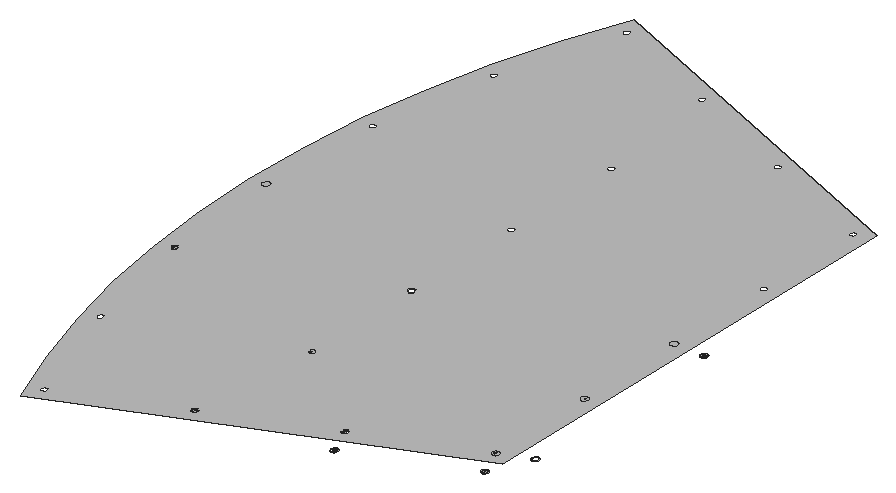
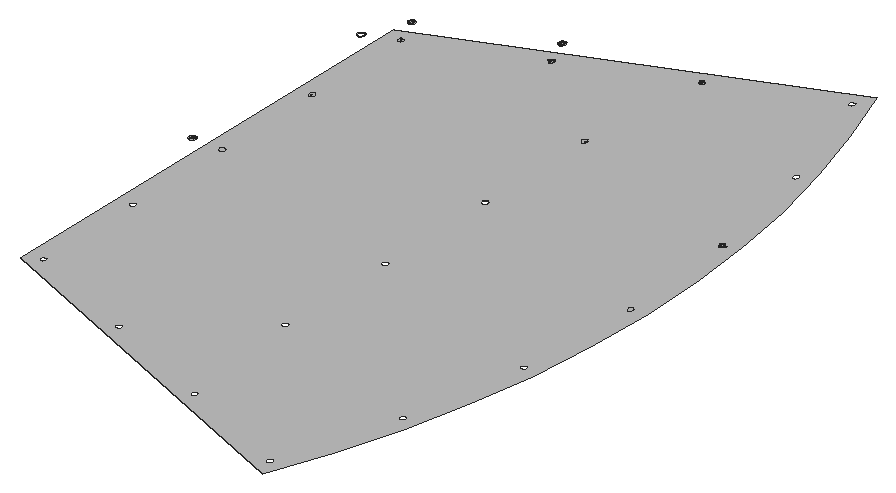
# SketchUp Ruby script. Lengths in inches.
U = 1.inch
M = Sketchup.active_model
def pt(a) = Geom::Point3d.new(a.map { |v| v * U })
def face(e, loops, mat)
  f = e.add_face(loops[0].map { |a| pt(a) })
  loops[1..].each { |l| e.add_face(l.map { |a| pt(a) }).erase! }
  f.material = f.back_material = mat if mat
  f
end
# faces: each face lists its corners as indices into pts; further lists are holes
def faces(e, pts, list, mat = nil) = list.each { |f| face(e, (f[0].is_a?(Array) ? f : [f]).map { |l| l.map { |i| pts[i] } }, mat) }
# xy, xz, yz: faces in a plane at the given z, y or x. An outline is a flat list of corners, or four numbers for a rectangle; further outlines are holes
def ring(l) = l.size == 4 ? [[l[0], l[1]], [l[2], l[1]], [l[2], l[3]], [l[0], l[3]]] : l.each_slice(2).to_a
def flat(e, list, mat, &to3) = list.each { |f| face(e, (f[0].is_a?(Array) ? f : [f]).map { |l| ring(l).map { |u, v| to3.(u, v) } }, mat) }
def xy(e, z, list, mat = nil) = flat(e, list, mat) { |x, y| [x, y, z] }
def xz(e, y, list, mat = nil) = flat(e, list, mat) { |x, z| [x, y, z] }
def yz(e, x, list, mat = nil) = flat(e, list, mat) { |y, z| [x, y, z] }
def lines(e, pts, list) = list.each { |a, b| e.add_line(pt(pts[a]), pt(pts[b])) }
# prism: a flat outline (further loops are holes) pulled along v
def prism(e, loops, v, mat = nil)
  f = face(e, loops, mat); d = Geom::Vector3d.new(v.map { |x| x * U })
  f.pushpull(f.normal.samedirection?(d) ? d.length : -d.length)
end
def box(e, o, s, mat = nil) = prism(e, [[o, [o[0] + s[0], o[1], o[2]], [o[0] + s[0], o[1] + s[1], o[2]], [o[0], o[1] + s[1], o[2]]]], [0, 0, s[2]], mat)
def at(x, y, z, deg = 0) = Geom::Transformation.translation(pt([x, y, z])) * Geom::Transformation.rotation(ORIGIN, Z_AXIS, deg.degrees)
def axes(o, x, y, z) = Geom::Transformation.new([*x, 0, *y, 0, *z, 0, *pt(o).to_a, 1])
def part(name) = M.definitions.add(name)
# library, detail: a bought-in or finely detailed component or shape, given as its bounding box
def library(name, o, s) = part(name).tap { |d| box(d.entities, o, s) }
def detail(e, o, s) = box(e.add_group.entities, o, s)
def put(e, d, t, mat = nil) = e.add_instance(d, t).tap { |i| i.material = mat if mat }
def group(e, t, mat = nil) = e.add_group.tap { |g| g.transformation = t; g.material = mat if mat }.entities
root = M.entities
M.materials.add("[Metal_Steel_Textured_White]").color = [191, 191, 191]
xy(root,3.625,[[[125.229,153.192,124.616,154.822,124.11,156.489,123.715,158.185,123.431,159.904,123.26,161.637,123.203,163.377,123.26,165.118,123.431,166.851,123.715,168.57,124.11,170.266,124.616,171.932,125.229,173.5625,134.847,169.578,134.847,157.176],[125.448,172.951,125.471,172.954,125.493,172.963,125.511,172.977,125.525,172.995,125.534,173.017,125.537,173.04,125.534,173.0625,125.525,173.084,125.511,173.102,125.493,173.117,125.471,173.125,125.448,173.128,125.425,173.125,125.404,173.117,125.385,173.102,125.371,173.084,125.362,173.0625,125.359,173.04,125.362,173.017,125.371,172.995,125.385,172.977,125.404,172.963,125.425,172.954],[134.448,163.289,134.471,163.292,134.492,163.3,134.511,163.315,134.525,163.333,134.534,163.354,134.537,163.377,134.534,163.4,134.525,163.422,134.511,163.44,134.492,163.454,134.471,163.463,134.448,163.466,134.425,163.463,134.404,163.454,134.385,163.44,134.371,163.422,134.362,163.4,134.359,163.377,134.362,163.354,134.371,163.333,134.385,163.315,134.404,163.3,134.425,163.292],[124.428,156.761,124.451,156.764,124.473,156.773,124.491,156.787,124.505,156.805,124.514,156.827,124.517,156.85,124.514,156.873,124.505,156.894,124.491,156.913,124.473,156.927,124.451,156.936,124.428,156.939,124.405,156.936,124.384,156.927,124.365,156.913,124.351,156.894,124.342,156.873,124.339,156.85,124.342,156.827,124.351,156.805,124.365,156.787,124.384,156.773,124.405,156.764],[134.448,157.354,134.471,157.357,134.492,157.366,134.511,157.38,134.525,157.399,134.534,157.42,134.537,157.443,134.534,157.466,134.525,157.488,134.511,157.506,134.492,157.52,134.471,157.529,134.448,157.532,134.425,157.529,134.404,157.52,134.385,157.506,134.371,157.488,134.362,157.466,134.359,157.443,134.362,157.42,134.371,157.399,134.385,157.38,134.404,157.366,134.425,157.357],[123.81,166.578,123.833,166.581,123.854,166.59,123.873,166.604,123.887,166.623,123.896,166.644,123.899,166.667,123.896,166.69,123.887,166.712,123.873,166.73,123.854,166.744,123.833,166.753,123.81,166.756,123.787,166.753,123.765,166.744,123.747,166.73,123.733,166.712,123.724,166.69,123.721,166.667,123.724,166.644,123.733,166.623,123.747,166.604,123.765,166.59,123.787,166.581],[128.448,154.869,128.471,154.872,128.493,154.881,128.511,154.895,128.525,154.913,128.534,154.935,128.537,154.958,128.534,154.981,128.525,155.002,128.511,155.021,128.493,155.035,128.471,155.044,128.448,155.047,128.425,155.044,128.404,155.035,128.385,155.021,128.371,155.002,128.362,154.981,128.359,154.958,128.362,154.935,128.371,154.913,128.385,154.895,128.404,154.881,128.425,154.872],[123.603,163.289,123.626,163.292,123.647,163.3,123.665,163.315,123.68,163.333,123.688,163.354,123.691,163.377,123.688,163.4,123.68,163.422,123.665,163.44,123.647,163.454,123.626,163.463,123.603,163.466,123.58,163.463,123.558,163.454,123.54,163.44,123.526,163.422,123.517,163.4,123.514,163.377,123.517,163.354,123.526,163.333,123.54,163.315,123.558,163.3,123.58,163.292],[125.448,153.626,125.471,153.629,125.493,153.638,125.511,153.652,125.525,153.671,125.534,153.692,125.537,153.715,125.534,153.738,125.525,153.76,125.511,153.778,125.493,153.792,125.471,153.801,125.448,153.804,125.425,153.801,125.404,153.792,125.385,153.778,125.371,153.76,125.362,153.738,125.359,153.715,125.362,153.692,125.371,153.671,125.385,153.652,125.404,153.638,125.425,153.629],[128.792,164.944,128.815,164.947,128.837,164.956,128.855,164.97,128.869,164.988,128.878,165.01,128.881,165.033,128.878,165.056,128.869,165.077,128.855,165.096,128.837,165.11,128.815,165.119,128.792,165.122,128.769,165.119,128.748,165.11,128.73,165.096,128.715,165.077,128.707,165.056,128.704,165.033,128.707,165.01,128.715,164.988,128.73,164.97,128.748,164.956,128.769,164.947],[128.792,158.322,128.815,158.325,128.837,158.334,128.855,158.348,128.869,158.367,128.878,158.388,128.881,158.411,128.878,158.434,128.869,158.456,128.855,158.474,128.837,158.488,128.815,158.497,128.792,158.5,128.769,158.497,128.748,158.488,128.73,158.474,128.715,158.456,128.707,158.434,128.704,158.411,128.707,158.388,128.715,158.367,128.73,158.348,128.748,158.334,128.769,158.325],[131.448,170.465,131.471,170.468,131.492,170.477,131.511,170.492,131.525,170.51,131.534,170.531,131.537,170.554,131.534,170.577,131.525,170.599,131.511,170.617,131.492,170.631,131.471,170.64,131.448,170.643,131.425,170.64,131.404,170.631,131.385,170.617,131.371,170.599,131.362,170.577,131.359,170.554,131.362,170.531,131.371,170.51,131.385,170.492,131.404,170.477,131.425,170.468],[134.448,160.321,134.471,160.324,134.492,160.333,134.511,160.347,134.525,160.366,134.534,160.387,134.537,160.41,134.534,160.433,134.525,160.455,134.511,160.473,134.492,160.487,134.471,160.496,134.448,160.499,134.425,160.496,134.404,160.487,134.385,160.473,134.371,160.455,134.362,160.433,134.359,160.41,134.362,160.387,134.371,160.366,134.385,160.347,134.404,160.333,134.425,160.324],[124.428,169.816,124.451,169.819,124.473,169.828,124.491,169.842,124.505,169.861,124.514,169.882,124.517,169.905,124.514,169.928,124.505,169.949,124.491,169.968,124.473,169.982,124.451,169.991,124.428,169.994,124.405,169.991,124.384,169.982,124.365,169.968,124.351,169.949,124.342,169.928,124.339,169.905,124.342,169.882,124.351,169.861,124.365,169.842,124.384,169.828,124.405,169.819],[128.792,168.255,128.815,168.258,128.837,168.267,128.855,168.281,128.869,168.299,128.878,168.321,128.881,168.344,128.878,168.367,128.869,168.388,128.855,168.406,128.837,168.421,128.815,168.429,128.792,168.432,128.769,168.429,128.748,168.421,128.73,168.406,128.715,168.388,128.707,168.367,128.704,168.344,128.707,168.321,128.715,168.299,128.73,168.281,128.748,168.267,128.769,168.258],[134.448,166.256,134.471,166.259,134.492,166.268,134.511,166.282,134.525,166.3,134.534,166.322,134.537,166.345,134.534,166.368,134.525,166.389,134.511,166.407,134.492,166.422,134.471,166.43,134.448,166.433,134.425,166.43,134.404,166.422,134.385,166.407,134.371,166.389,134.362,166.368,134.359,166.345,134.362,166.322,134.371,166.3,134.385,166.282,134.404,166.268,134.425,166.259],[123.81,159.999,123.833,160.002,123.854,160.011,123.873,160.025,123.887,160.043,123.896,160.065,123.899,160.088,123.896,160.111,123.887,160.132,123.873,160.15,123.854,160.165,123.833,160.173,123.81,160.177,123.787,160.173,123.765,160.165,123.747,160.15,123.733,160.132,123.724,160.111,123.721,160.088,123.724,160.065,123.733,160.043,123.747,160.025,123.765,160.011,123.787,160.002],[128.448,171.708,128.471,171.711,128.493,171.72,128.511,171.734,128.525,171.753,128.534,171.774,128.537,171.797,128.534,171.82,128.525,171.841,128.511,171.86,128.493,171.874,128.471,171.883,128.448,171.886,128.425,171.883,128.404,171.874,128.385,171.86,128.371,171.841,128.362,171.82,128.359,171.797,128.362,171.774,128.371,171.753,128.385,171.734,128.404,171.72,128.425,171.711],[134.448,169.223,134.471,169.226,134.492,169.235,134.511,169.249,134.525,169.267,134.534,169.289,134.537,169.312,134.534,169.335,134.525,169.356,134.511,169.375,134.492,169.389,134.471,169.398,134.448,169.401,134.425,169.398,134.404,169.389,134.385,169.375,134.371,169.356,134.362,169.335,134.359,169.312,134.362,169.289,134.371,169.267,134.385,169.249,134.404,169.235,134.425,169.226],[131.448,156.112,131.471,156.115,131.492,156.124,131.511,156.138,131.525,156.156,131.534,156.177,131.537,156.2,131.534,156.223,131.525,156.245,131.511,156.263,131.492,156.277,131.471,156.286,131.448,156.289,131.425,156.286,131.404,156.277,131.385,156.263,131.371,156.245,131.362,156.223,131.359,156.2,131.362,156.177,131.371,156.156,131.385,156.138,131.404,156.124,131.425,156.115],[128.792,161.633,128.815,161.636,128.837,161.645,128.855,161.659,128.869,161.678,128.878,161.699,128.881,161.722,128.878,161.745,128.869,161.766,128.855,161.785,128.837,161.799,128.815,161.808,128.792,161.811,128.769,161.808,128.748,161.799,128.73,161.785,128.715,161.766,128.707,161.745,128.704,161.722,128.707,161.699,128.715,161.678,128.73,161.659,128.748,161.645,128.769,161.636]],[[128.448,154.869,128.425,154.872,128.404,154.881,128.385,154.895,128.371,154.913,128.362,154.935,128.359,154.958,128.362,154.981,128.371,155.002,128.385,155.021,128.404,155.035,128.425,155.044,128.448,155.047,128.471,155.044,128.493,155.035,128.511,155.021,128.525,155.002,128.534,154.981,128.537,154.958,128.534,154.935,128.525,154.913,128.511,154.895,128.493,154.881,128.471,154.872],[128.448,154.87,128.471,154.873,128.492,154.882,128.51,154.896,128.524,154.914,128.533,154.935,128.536,154.958,128.533,154.981,128.524,155.002,128.51,155.02,128.492,155.034,128.471,155.043,128.448,155.046,128.425,155.043,128.404,155.034,128.386,155.02,128.372,155.002,128.363,154.981,128.36,154.958,128.363,154.935,128.372,154.914,128.386,154.896,128.404,154.882,128.425,154.873]],[[128.448,154.921,128.439,154.923,128.43,154.926,128.422,154.932,128.416,154.94,128.413,154.948,128.411,154.958,128.413,154.967,128.416,154.976,128.422,154.984,128.43,154.99,128.439,154.993,128.448,154.994,128.458,154.993,128.466,154.99,128.474,154.984,128.48,154.976,128.483,154.967,128.485,154.958,128.483,154.948,128.48,154.94,128.474,154.932,128.466,154.926,128.458,154.923],[128.448,154.938,128.453,154.939,128.458,154.941,128.462,154.944,128.465,154.948,128.467,154.953,128.468,154.958,128.467,154.963,128.465,154.968,128.462,154.972,128.458,154.975,128.453,154.977,128.448,154.978,128.443,154.977,128.438,154.975,128.434,154.972,128.431,154.968,128.429,154.963,128.428,154.958,128.429,154.953,128.431,154.948,128.434,154.944,128.438,154.941,128.443,154.939]],[128.448,154.938,128.443,154.939,128.438,154.941,128.434,154.944,128.431,154.948,128.429,154.953,128.428,154.958,128.429,154.963,128.431,154.968,128.434,154.972,128.438,154.975,128.443,154.977,128.448,154.978,128.453,154.977,128.458,154.975,128.462,154.972,128.465,154.968,128.467,154.963,128.468,154.958,128.467,154.953,128.465,154.948,128.462,154.944,128.458,154.941,128.453,154.939],[[131.754,155.374,131.731,155.377,131.709,155.386,131.691,155.4,131.677,155.418,131.668,155.44,131.665,155.463,131.668,155.486,131.677,155.507,131.691,155.526,131.709,155.54,131.731,155.549,131.754,155.552,131.777,155.549,131.798,155.54,131.816,155.526,131.831,155.507,131.839,155.486,131.842,155.463,131.839,155.44,131.831,155.418,131.816,155.4,131.798,155.386,131.777,155.377],[131.754,155.375,131.776,155.378,131.798,155.387,131.816,155.401,131.83,155.419,131.839,155.44,131.842,155.463,131.839,155.486,131.83,155.507,131.816,155.525,131.798,155.539,131.776,155.548,131.754,155.551,131.731,155.548,131.71,155.539,131.691,155.525,131.677,155.507,131.669,155.486,131.666,155.463,131.669,155.44,131.677,155.419,131.691,155.401,131.71,155.387,131.731,155.378]],
  [[131.754,155.426,131.744,155.427,131.735,155.431,131.728,155.437,131.722,155.445,131.718,155.453,131.717,155.463,131.718,155.472,131.722,155.481,131.728,155.489,131.735,155.495,131.744,155.498,131.754,155.499,131.763,155.498,131.772,155.495,131.779,155.489,131.785,155.481,131.789,155.472,131.79,155.463,131.789,155.453,131.785,155.445,131.779,155.437,131.772,155.431,131.763,155.427],[131.754,155.443,131.759,155.444,131.764,155.446,131.768,155.449,131.771,155.453,131.773,155.458,131.774,155.463,131.773,155.468,131.771,155.473,131.768,155.477,131.764,155.48,131.759,155.482,131.754,155.483,131.748,155.482,131.744,155.48,131.739,155.477,131.736,155.473,131.734,155.468,131.734,155.458,131.736,155.453,131.739,155.449,131.744,155.446,131.748,155.444]],[131.754,155.443,131.748,155.444,131.744,155.446,131.739,155.449,131.736,155.453,131.734,155.458,131.734,155.468,131.736,155.473,131.739,155.477,131.744,155.48,131.748,155.482,131.754,155.483,131.759,155.482,131.764,155.48,131.768,155.477,131.771,155.473,131.773,155.468,131.774,155.463,131.773,155.458,131.771,155.453,131.768,155.449,131.764,155.446,131.759,155.444],[[131.448,156.112,131.425,156.115,131.404,156.124,131.385,156.138,131.371,156.156,131.362,156.177,131.359,156.2,131.362,156.223,131.371,156.245,131.385,156.263,131.404,156.277,131.425,156.286,131.448,156.289,131.471,156.286,131.492,156.277,131.511,156.263,131.525,156.245,131.534,156.223,131.537,156.2,131.534,156.177,131.525,156.156,131.511,156.138,131.492,156.124,131.471,156.115],[131.448,156.113,131.471,156.116,131.492,156.124,131.51,156.138,131.524,156.157,131.533,156.178,131.536,156.2,131.533,156.223,131.524,156.244,131.51,156.263,131.492,156.277,131.471,156.285,131.448,156.288,131.425,156.285,131.404,156.277,131.386,156.263,131.372,156.244,131.363,156.223,131.36,156.2,131.363,156.178,131.372,156.157,131.386,156.138,131.404,156.124,131.425,156.116]],[[131.448,156.164,131.439,156.165,131.43,156.169,131.422,156.175,131.416,156.182,131.413,156.191,131.411,156.2,131.413,156.21,131.416,156.219,131.422,156.226,131.43,156.232,131.439,156.236,131.448,156.237,131.458,156.236,131.466,156.232,131.474,156.226,131.48,156.219,131.483,156.21,131.485,156.2,131.483,156.191,131.48,156.182,131.474,156.175,131.466,156.169,131.458,156.165],[131.443,156.181,131.453,156.181,131.458,156.183,131.462,156.186,131.465,156.191,131.467,156.195,131.468,156.2,131.467,156.206,131.465,156.21,131.462,156.215,131.458,156.218,131.453,156.22,131.443,156.22,131.438,156.218,131.434,156.215,131.431,156.21,131.429,156.206,131.428,156.2,131.429,156.195,131.431,156.191,131.434,156.186,131.438,156.183]],[131.443,156.181,131.438,156.183,131.434,156.186,131.431,156.191,131.429,156.195,131.428,156.2,131.429,156.206,131.431,156.21,131.434,156.215,131.438,156.218,131.443,156.22,131.453,156.22,131.458,156.218,131.462,156.215,131.465,156.21,131.467,156.206,131.468,156.2,131.467,156.195,131.465,156.191,131.462,156.186,131.458,156.183,131.453,156.181],
  [[134.754,156.617,134.731,156.62,134.709,156.628,134.691,156.643,134.677,156.661,134.668,156.682,134.665,156.705,134.668,156.728,134.677,156.75,134.691,156.768,134.709,156.782,134.731,156.791,134.754,156.794,134.777,156.791,134.798,156.782,134.816,156.768,134.831,156.75,134.839,156.728,134.842,156.705,134.839,156.682,134.831,156.661,134.816,156.643,134.798,156.628,134.777,156.62],[134.754,156.618,134.776,156.621,134.798,156.629,134.816,156.643,134.83,156.661,134.838,156.683,134.841,156.705,134.838,156.728,134.83,156.749,134.816,156.768,134.798,156.782,134.776,156.79,134.754,156.793,134.731,156.79,134.71,156.782,134.691,156.768,134.677,156.749,134.669,156.728,134.666,156.705,134.669,156.683,134.677,156.661,134.691,156.643,134.71,156.629,134.731,156.621]],[[134.754,156.669,134.744,156.67,134.735,156.674,134.728,156.68,134.722,156.687,134.718,156.696,134.717,156.705,134.718,156.715,134.722,156.724,134.728,156.731,134.735,156.737,134.744,156.741,134.754,156.742,134.763,156.741,134.772,156.737,134.779,156.731,134.785,156.724,134.789,156.715,134.79,156.705,134.789,156.696,134.785,156.687,134.779,156.68,134.772,156.674,134.763,156.67],[134.754,156.685,134.759,156.686,134.764,156.688,134.768,156.691,134.771,156.695,134.773,156.7,134.773,156.711,134.771,156.715,134.768,156.72,134.764,156.723,134.759,156.725,134.748,156.725,134.744,156.723,134.739,156.72,134.736,156.715,134.734,156.711,134.734,156.7,134.736,156.695,134.739,156.691,134.744,156.688,134.748,156.686]],[134.754,156.685,134.748,156.686,134.744,156.688,134.739,156.691,134.736,156.695,134.734,156.7,134.734,156.711,134.736,156.715,134.739,156.72,134.744,156.723,134.748,156.725,134.759,156.725,134.764,156.723,134.768,156.72,134.771,156.715,134.773,156.711,134.773,156.7,134.771,156.695,134.768,156.691,134.764,156.688,134.759,156.686],[[134.448,157.355,134.425,157.358,134.404,157.367,134.386,157.381,134.372,157.399,134.363,157.42,134.36,157.443,134.363,157.466,134.372,157.487,134.386,157.505,134.404,157.519,134.425,157.528,134.448,157.531,134.471,157.528,134.492,157.519,134.51,157.505,134.524,157.487,134.533,157.466,134.536,157.443,134.533,157.42,134.524,157.399,134.51,157.381,134.492,157.367,134.471,157.358],[134.448,157.407,134.457,157.408,134.466,157.411,134.474,157.417,134.48,157.425,134.483,157.434,134.485,157.443,134.483,157.453,134.48,157.461,134.474,157.469,134.466,157.475,134.457,157.478,134.448,157.48,134.439,157.478,134.43,157.475,134.422,157.469,134.416,157.461,134.413,157.453,134.411,157.443,134.413,157.434,134.416,157.425,134.422,157.417,134.43,157.411,134.439,157.408]],[[134.448,157.407,134.439,157.408,134.43,157.411,134.422,157.417,134.416,157.425,134.413,157.434,134.411,157.443,134.413,157.453,134.416,157.461,134.422,157.469,134.43,157.475,134.439,157.478,134.448,157.48,134.457,157.478,134.466,157.475,134.474,157.469,134.48,157.461,134.483,157.453,134.485,157.443,134.483,157.434,134.48,157.425,134.474,157.417,134.466,157.411,134.457,157.408],[134.448,157.423,134.453,157.424,134.458,157.426,134.462,157.429,134.465,157.433,134.467,157.438,134.468,157.443,134.467,157.448,134.465,157.453,134.462,157.457,134.458,157.46,134.453,157.462,134.448,157.463,134.443,157.462,134.438,157.46,134.434,157.457,134.431,157.453,134.429,157.448,134.428,157.443,134.429,157.438,134.431,157.433,134.434,157.429,134.438,157.426,134.443,157.424]],
  [134.448,157.423,134.443,157.424,134.438,157.426,134.434,157.429,134.431,157.433,134.429,157.438,134.428,157.443,134.429,157.448,134.431,157.453,134.434,157.457,134.438,157.46,134.443,157.462,134.448,157.463,134.453,157.462,134.458,157.46,134.462,157.457,134.465,157.453,134.467,157.448,134.468,157.443,134.467,157.438,134.465,157.433,134.462,157.429,134.458,157.426,134.453,157.424],[[135.246,157.685,135.223,157.688,135.202,157.697,135.184,157.711,135.169,157.729,135.161,157.751,135.158,157.774,135.161,157.797,135.169,157.818,135.184,157.837,135.202,157.851,135.223,157.86,135.246,157.863,135.269,157.86,135.291,157.851,135.309,157.837,135.323,157.818,135.332,157.797,135.335,157.774,135.332,157.751,135.323,157.729,135.309,157.711,135.291,157.697,135.269,157.688],[135.246,157.686,135.269,157.689,135.29,157.698,135.309,157.712,135.323,157.73,135.331,157.751,135.334,157.774,135.331,157.797,135.323,157.818,135.309,157.836,135.29,157.85,135.269,157.859,135.246,157.862,135.224,157.859,135.202,157.85,135.184,157.836,135.17,157.818,135.161,157.797,135.159,157.774,135.161,157.751,135.17,157.73,135.184,157.712,135.202,157.698,135.224,157.689]],[[128.792,158.323,128.77,158.326,128.748,158.335,128.73,158.349,128.716,158.367,128.707,158.389,128.704,158.411,128.707,158.434,128.716,158.455,128.73,158.473,128.748,158.487,128.77,158.496,128.792,158.499,128.815,158.496,128.836,158.487,128.855,158.473,128.869,158.455,128.877,158.434,128.88,158.411,128.877,158.389,128.869,158.367,128.855,158.349,128.836,158.335,128.815,158.326],[128.792,158.375,128.802,158.376,128.811,158.38,128.818,158.385,128.824,158.393,128.828,158.402,128.829,158.411,128.828,158.421,128.824,158.43,128.818,158.437,128.811,158.443,128.802,158.447,128.792,158.448,128.783,158.447,128.774,158.443,128.767,158.437,128.761,158.43,128.757,158.421,128.756,158.411,128.757,158.402,128.761,158.393,128.767,158.385,128.774,158.38,128.783,158.376]],[[123.81,159.999,123.787,160.002,123.765,160.011,123.747,160.025,123.733,160.043,123.724,160.065,123.721,160.088,123.724,160.111,123.733,160.132,123.747,160.15,123.765,160.165,123.787,160.173,123.81,160.177,123.833,160.173,123.854,160.165,123.873,160.15,123.887,160.132,123.896,160.111,123.899,160.088,123.896,160.065,123.887,160.043,123.873,160.025,123.854,160.011,123.833,160.002],[123.81,160,123.833,160.003,123.854,160.011,123.872,160.025,123.886,160.044,123.895,160.065,123.898,160.088,123.895,160.11,123.886,160.132,123.872,160.15,123.854,160.164,123.833,160.173,123.81,160.176,123.787,160.173,123.766,160.164,123.748,160.15,123.734,160.132,123.725,160.11,123.722,160.088,123.725,160.065,123.734,160.044,123.748,160.025,123.766,160.011,123.787,160.003]],[[123.81,160.051,123.8,160.052,123.792,160.056,123.784,160.062,123.778,160.069,123.774,160.078,123.773,160.088,123.774,160.097,123.778,160.106,123.784,160.113,123.792,160.119,123.8,160.123,123.81,160.124,123.819,160.123,123.828,160.119,123.836,160.113,123.841,160.106,123.845,160.097,123.846,160.088,123.845,160.078,123.841,160.069,123.836,160.062,123.828,160.056,123.819,160.052],[123.805,160.068,123.815,160.068,123.82,160.07,123.824,160.074,123.827,160.078,123.829,160.082,123.83,160.088,123.829,160.093,123.827,160.098,123.824,160.102,123.82,160.105,123.815,160.107,123.81,160.108,123.805,160.107,123.8,160.105,123.796,160.102,123.793,160.098,123.791,160.093,123.79,160.088,123.791,160.082,123.793,160.078,123.796,160.074,123.8,160.07]],
  [123.805,160.068,123.8,160.07,123.796,160.074,123.793,160.078,123.791,160.082,123.79,160.088,123.791,160.093,123.793,160.098,123.796,160.102,123.8,160.105,123.805,160.107,123.81,160.108,123.815,160.107,123.82,160.105,123.824,160.102,123.827,160.098,123.829,160.093,123.83,160.088,123.829,160.082,123.827,160.078,123.824,160.074,123.82,160.07,123.815,160.068],[[134.448,160.322,134.425,160.325,134.404,160.334,134.386,160.348,134.372,160.366,134.363,160.388,134.36,160.41,134.363,160.433,134.372,160.454,134.386,160.472,134.404,160.486,134.425,160.495,134.448,160.498,134.471,160.495,134.492,160.486,134.51,160.472,134.524,160.454,134.533,160.433,134.536,160.41,134.533,160.388,134.524,160.366,134.51,160.348,134.492,160.334,134.471,160.325],[134.448,160.374,134.457,160.375,134.466,160.379,134.474,160.384,134.48,160.392,134.483,160.401,134.485,160.41,134.483,160.42,134.48,160.429,134.474,160.436,134.466,160.442,134.457,160.446,134.448,160.447,134.439,160.446,134.43,160.442,134.422,160.436,134.416,160.429,134.413,160.42,134.411,160.41,134.413,160.401,134.416,160.392,134.422,160.384,134.43,160.379,134.439,160.375]],[[128.792,161.633,128.769,161.636,128.748,161.645,128.73,161.659,128.715,161.678,128.707,161.699,128.704,161.722,128.707,161.745,128.715,161.766,128.73,161.785,128.748,161.799,128.769,161.808,128.792,161.811,128.815,161.808,128.837,161.799,128.855,161.785,128.869,161.766,128.878,161.745,128.881,161.722,128.878,161.699,128.869,161.678,128.855,161.659,128.837,161.645,128.815,161.636],[128.792,161.634,128.815,161.637,128.836,161.646,128.855,161.66,128.869,161.678,128.877,161.699,128.88,161.722,128.877,161.745,128.869,161.766,128.855,161.784,128.836,161.798,128.815,161.807,128.792,161.81,128.77,161.807,128.748,161.798,128.73,161.784,128.716,161.766,128.707,161.745,128.704,161.722,128.707,161.699,128.716,161.678,128.73,161.66,128.748,161.646,128.77,161.637]],[[123.603,163.289,123.58,163.292,123.559,163.301,123.54,163.315,123.526,163.333,123.518,163.355,123.515,163.377,123.514,163.377,123.517,163.4,123.526,163.422,123.54,163.44,123.558,163.454,123.58,163.463,123.603,163.466,123.626,163.463,123.647,163.454,123.665,163.44,123.68,163.422,123.688,163.4,123.691,163.377,123.69,163.377,123.6875,163.355,123.679,163.333,123.665,163.315,123.647,163.301,123.625,163.292],[123.603,163.341,123.612,163.342,123.621,163.346,123.628,163.352,123.634,163.359,123.638,163.368,123.639,163.377,123.623,163.377,123.622,163.372,123.62,163.367,123.617,163.363,123.613,163.36,123.608,163.358,123.603,163.357,123.597,163.358,123.593,163.36,123.588,163.363,123.585,163.367,123.583,163.372,123.583,163.377,123.566,163.377,123.567,163.368,123.571,163.359,123.577,163.352,123.584,163.346,123.593,163.342],[123.583,163.377,123.623,163.377,123.622,163.383,123.62,163.387,123.617,163.392,123.613,163.395,123.608,163.397,123.597,163.397,123.593,163.395,123.588,163.392,123.585,163.387,123.583,163.383]],[[134.448,163.289,134.425,163.292,134.404,163.3,134.385,163.315,134.371,163.333,134.362,163.354,134.359,163.377,134.36,163.377,134.363,163.4,134.372,163.421,134.386,163.44,134.404,163.454,134.425,163.462,134.448,163.465,134.471,163.462,134.492,163.454,134.51,163.44,134.524,163.421,134.533,163.4,134.536,163.377,134.537,163.377,134.534,163.354,134.525,163.333,134.511,163.315,134.492,163.3,134.471,163.292],[134.448,163.357,134.453,163.358,134.458,163.36,134.462,163.363,134.465,163.367,134.467,163.372,134.468,163.377,134.485,163.377,134.483,163.387,134.48,163.396,134.474,163.403,134.466,163.409,134.457,163.413,134.448,163.414,134.439,163.413,134.43,163.409,134.422,163.403,134.416,163.396,134.413,163.387,134.411,163.377,134.428,163.377,134.429,163.372,134.431,163.367,134.434,163.363,134.438,163.36,134.443,163.358],[134.428,163.377,134.468,163.377,134.467,163.383,134.465,163.387,134.462,163.392,134.458,163.395,134.453,163.397,134.443,163.397,134.438,163.395,134.434,163.392,134.431,163.387,134.429,163.383]],
  [135.246,163.289,135.223,163.292,135.202,163.3,135.184,163.315,135.169,163.333,135.161,163.354,135.158,163.377,135.159,163.377,135.161,163.355,135.17,163.333,135.184,163.315,135.202,163.301,135.224,163.292,135.246,163.289,135.269,163.292,135.29,163.301,135.309,163.315,135.323,163.333,135.331,163.355,135.334,163.377,135.335,163.377,135.332,163.354,135.323,163.333,135.309,163.315,135.291,163.3,135.269,163.292],[135.246,163.289,135.224,163.292,135.202,163.301,135.184,163.315,135.17,163.333,135.161,163.355,135.159,163.377,135.21,163.377,135.211,163.368,135.215,163.359,135.221,163.352,135.228,163.346,135.237,163.342,135.246,163.341,135.256,163.342,135.265,163.346,135.272,163.352,135.278,163.359,135.282,163.368,135.283,163.377,135.334,163.377,135.331,163.355,135.323,163.333,135.309,163.315,135.29,163.301,135.269,163.292],[135.246,163.341,135.237,163.342,135.228,163.346,135.221,163.352,135.215,163.359,135.211,163.368,135.21,163.377,135.226,163.377,135.227,163.372,135.229,163.367,135.232,163.363,135.236,163.36,135.241,163.358,135.246,163.357,135.252,163.358,135.256,163.36,135.261,163.363,135.264,163.367,135.266,163.372,135.266,163.377,135.283,163.377,135.282,163.368,135.278,163.359,135.272,163.352,135.265,163.346,135.256,163.342],[135.246,163.357,135.241,163.358,135.236,163.36,135.232,163.363,135.229,163.367,135.227,163.372,135.226,163.377,135.266,163.377,135.266,163.372,135.264,163.367,135.261,163.363,135.256,163.36,135.252,163.358],[135.158,163.377,135.161,163.4,135.169,163.422,135.184,163.44,135.202,163.454,135.223,163.463,135.246,163.466,135.269,163.463,135.291,163.454,135.309,163.44,135.323,163.422,135.332,163.4,135.335,163.377,135.334,163.377,135.331,163.4,135.323,163.421,135.309,163.44,135.29,163.454,135.269,163.462,135.246,163.465,135.224,163.462,135.202,163.454,135.184,163.44,135.17,163.421,135.161,163.4,135.159,163.377],
  [135.159,163.377,135.161,163.4,135.17,163.421,135.184,163.44,135.202,163.454,135.224,163.462,135.246,163.465,135.269,163.462,135.29,163.454,135.309,163.44,135.323,163.421,135.331,163.4,135.334,163.377,135.283,163.377,135.282,163.387,135.278,163.396,135.272,163.403,135.265,163.409,135.256,163.413,135.246,163.414,135.237,163.413,135.228,163.409,135.221,163.403,135.215,163.396,135.211,163.387,135.21,163.377],[135.21,163.377,135.211,163.387,135.215,163.396,135.221,163.403,135.228,163.409,135.237,163.413,135.246,163.414,135.256,163.413,135.265,163.409,135.272,163.403,135.278,163.396,135.282,163.387,135.283,163.377,135.266,163.377,135.266,163.383,135.264,163.387,135.261,163.392,135.256,163.395,135.252,163.397,135.241,163.397,135.236,163.395,135.232,163.392,135.229,163.387,135.227,163.383,135.226,163.377],[135.226,163.377,135.227,163.383,135.229,163.387,135.232,163.392,135.236,163.395,135.241,163.397,135.252,163.397,135.256,163.395,135.261,163.392,135.264,163.387,135.266,163.383,135.266,163.377]],"[Metal_Steel_Textured_White]")
